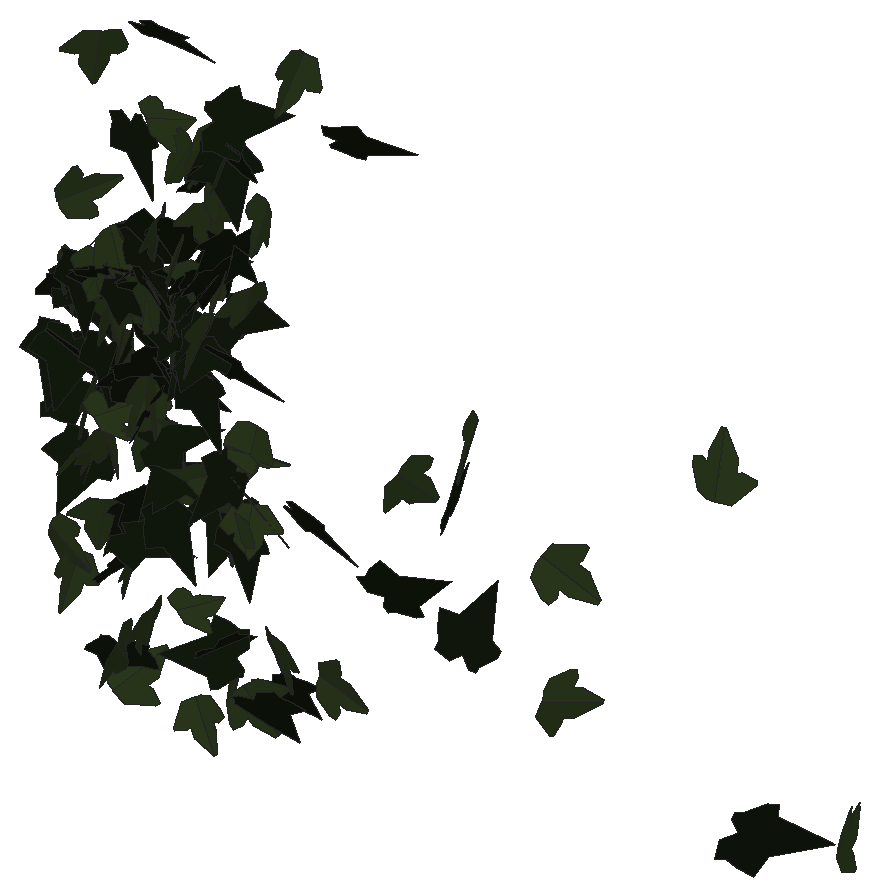
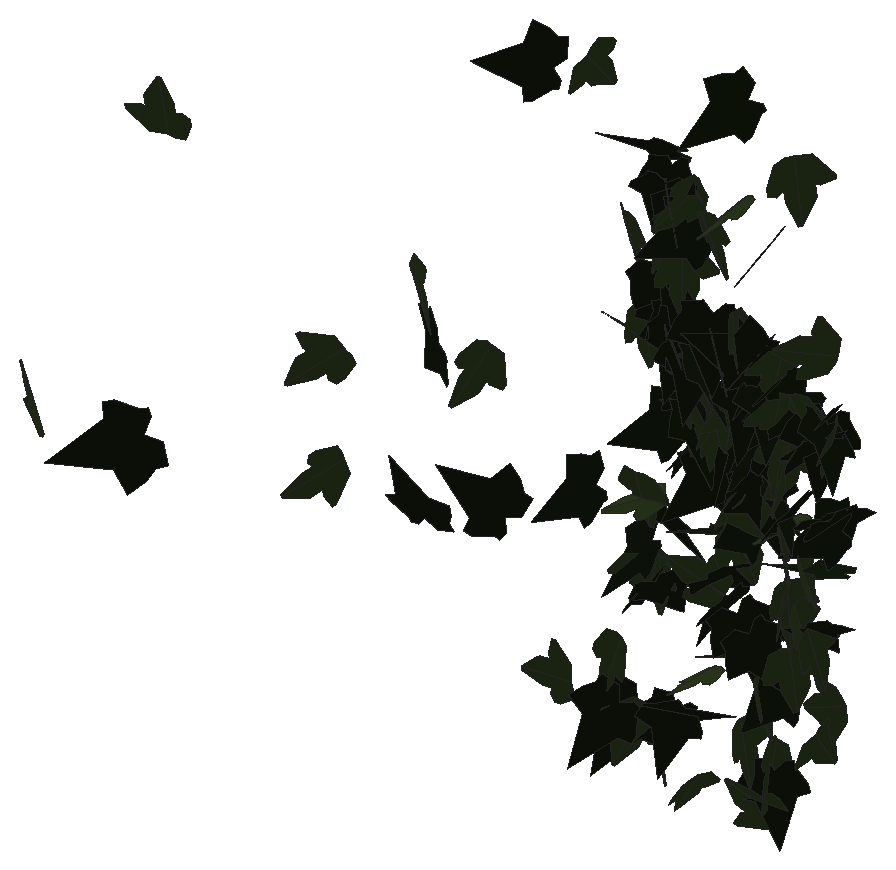
# SketchUp Ruby script. Lengths in inches.
U = 1.inch
M = Sketchup.active_model
def pt(a) = Geom::Point3d.new(a.map { |v| v * U })
def face(e, loops, mat)
  f = e.add_face(loops[0].map { |a| pt(a) })
  loops[1..].each { |l| e.add_face(l.map { |a| pt(a) }).erase! }
  f.material = f.back_material = mat if mat
  f
end
# faces: each face lists its corners as indices into pts; further lists are holes
def faces(e, pts, list, mat = nil) = list.each { |f| face(e, (f[0].is_a?(Array) ? f : [f]).map { |l| l.map { |i| pts[i] } }, mat) }
# xy, xz, yz: faces in a plane at the given z, y or x. An outline is a flat list of corners, or four numbers for a rectangle; further outlines are holes
def ring(l) = l.size == 4 ? [[l[0], l[1]], [l[2], l[1]], [l[2], l[3]], [l[0], l[3]]] : l.each_slice(2).to_a
def flat(e, list, mat, &to3) = list.each { |f| face(e, (f[0].is_a?(Array) ? f : [f]).map { |l| ring(l).map { |u, v| to3.(u, v) } }, mat) }
def xy(e, z, list, mat = nil) = flat(e, list, mat) { |x, y| [x, y, z] }
def xz(e, y, list, mat = nil) = flat(e, list, mat) { |x, z| [x, y, z] }
def yz(e, x, list, mat = nil) = flat(e, list, mat) { |y, z| [x, y, z] }
def lines(e, pts, list) = list.each { |a, b| e.add_line(pt(pts[a]), pt(pts[b])) }
# prism: a flat outline (further loops are holes) pulled along v
def prism(e, loops, v, mat = nil)
  f = face(e, loops, mat); d = Geom::Vector3d.new(v.map { |x| x * U })
  f.pushpull(f.normal.samedirection?(d) ? d.length : -d.length)
end
def box(e, o, s, mat = nil) = prism(e, [[o, [o[0] + s[0], o[1], o[2]], [o[0] + s[0], o[1] + s[1], o[2]], [o[0], o[1] + s[1], o[2]]]], [0, 0, s[2]], mat)
def at(x, y, z, deg = 0) = Geom::Transformation.translation(pt([x, y, z])) * Geom::Transformation.rotation(ORIGIN, Z_AXIS, deg.degrees)
def axes(o, x, y, z) = Geom::Transformation.new([*x, 0, *y, 0, *z, 0, *pt(o).to_a, 1])
def part(name) = M.definitions.add(name)
# library, detail: a bought-in or finely detailed component or shape, given as its bounding box
def library(name, o, s) = part(name).tap { |d| box(d.entities, o, s) }
def detail(e, o, s) = box(e.add_group.entities, o, s)
def put(e, d, t, mat = nil) = e.add_instance(d, t).tap { |i| i.material = mat if mat }
def group(e, t, mat = nil) = e.add_group.tap { |g| g.transformation = t; g.material = mat if mat }.entities
root = M.entities
M.materials.add("efeu1").color = [18, 25, 13]
M.materials.add("efeu2").color = [43, 57, 29]
c1 = part("ivyleaf_9")
p = [[1.54,2.16,1.25],[1.36,2.04,1.19],[-0.21,0.99,0.68],[-0.71,1.11,0.82],[-0.85,0.86,0.67],[-0.8,0.17,0.21],
  [-0.9,-0.01,0.1],[-0.67,-0.16,-0.02],[-0.08,-0.08,-0.05],[-0.03,-0.6,-0.4],[0.65,-0.88,-0.66],[0.83,-0.6,-0.49],
  [1.29,-0.42,-0.43],[1.8125,-0.07,-0.26],[1.21,0.44,0.15]]
faces(c1.entities,p,[[0,1,2,3,4,5,6,7,8,9,10,11,12,13,14]],"efeu1")
c2 = part("ivyleaf_10")
p = [[0,0.5,-0.03],[-0.0625,2.02,-0.43],[-0.19,2.01,-0.46],[-0.54,1.05,-0.29],[-0.52,0.625,-0.18],[-0.83,0.76,-0.28],
  [-1.16,0.64,-0.33],[-1.15,0.33,-0.24],[-0.77,-0.39,0.02],[-0.3,-0.51,0.16],[0.04,-0.48,0.23],[-0.02,2.01,-0.4375],
  [-0.06,2.01,-0.43],[0.04,-0.49,0.23],[0.67,-0.49,0.14],[1.38,0.36,-0.2],[1.375,0.51,-0.24],[0.81,0.65,-0.19],
  [0.62,0.59,-0.15],[0.6,1.09,-0.28],[0.5,1.23,-0.31]]
faces(c2.entities,p,[[0,1,2,3,4,5,6,7,8,9,10],[11,12,0,13,14,15,16,17,18,19,20]],"efeu2")
put(root,c1,axes([589.86,129.38,257.64],[-0.38156,-0.98328,-0.03529],[0.01021,0.03389,-1.05471],[0.98386,-0.38169,-0.00274]))
put(root,c1,axes([590.56,128.76,261.47],[-0.136,1.02686,0.32023],[-0.14631,0.30212,-1.03092],[-1.06564,-0.17253,0.10067]))
put(root,c2,axes([590.15,129.05,261.39],[-0.4513,0.99422,-0.05253],[-0.00038,-0.05785,-1.09158],[-0.9956,-0.45065,0.02423]))
put(root,c1,axes([589.49,129.37,257.3125],[1.00767,-0.24895,0.30361],[0.29888,-0.05592,-1.03783],[0.2546,1.05093,0.01669]))
put(root,c2,axes([590.42,129.98,252.09],[0.06529,-1.04507,0.14266],[0.00107,-0.14286,-1.04708],[1.05476,0.06483,-0.00777]))
put(root,c1,axes([590.3125,129.42,257.61],[-0.48859,-0.93303,-0.00792],[0.20269,-0.09741,-1.02896],[0.91078,-0.47885,0.22474]))
put(root,c1,axes([589.84,129,255.1],[0.95581,-0.42825,-0.09163],[0.37043,0.90792,-0.37927],[0.23362,0.31251,0.97629]))
put(root,c2,axes([590.58,129.38,247.28],[0.23753,0.84721,-0.56766],[-0.14143,-0.54986,-0.87982],[-1.00995,0.27625,-0.0103]))
put(root,c1,axes([590.76,129.91,252.54],[-0.71489,-0.78039,-0.02428],[0.12744,-0.08416,-1.04754],[0.7703,-0.71034,0.15078]))
put(root,c2,axes([590.11,128.87,248.73],[-0.43886,0.21107,-0.95915],[0.8493,-0.44597,-0.48674],[-0.49316,-0.95587,0.0153]))
put(root,c1,axes([590.99,128.35,261.39],[0.53183,0.9298,-0.32357],[-0.13362,-0.29619,-1.07074],[-0.97538,0.54755,-0.02974]))
put(root,c2,axes([590.9,129.92,255.37],[0.52404,-0.88255,0.26397],[0.14877,-0.21863,-1.02628],[0.90908,0.54451,0.01578]))
put(root,c2,axes([591.11,129.92,252.97],[0.28838,-1.01393,0.11412],[0.0212,-0.11261,-1.05409],[1.02011,0.28897,-0.01036]))
put(root,c2,axes([590.72,128.84,264.89],[-0.09538,-0.31554,1.0512],[0.34503,0.99305,0.32938],[-1.04189,0.35774,0.01285]))
put(root,c1,axes([590.61,129.5,261.02],[0.19183,-0.93138,-0.50614],[0.13029,0.53118,-0.92807],[1.05198,0.10405,0.20723]))
put(root,c1,axes([590.89,129.36,261.36],[0.16546,-1.04814,0.20582],[0.00088,-0.20814,-1.06066],[1.06815,0.16253,-0.03101]))
put(root,c2,axes([591.77,129.8,253.75],[-0.17683,-1.03716,-0.15633],[-0.01256,0.16062,-1.0514],[1.0488,-0.17295,-0.03895]))
put(root,c2,axes([592.03,129.375,250.38],[-0.75065,-0.73163,0.14522],[-0.08676,-0.11898,-1.04793],[0.74084,-0.75525,0.02442]))
put(root,c2,axes([592.0625,128.96,262.08],[1.00444,-0.14869,-0.34824],[-0.33329,0.12137,-1.01315],[0.17972,1.05614,0.0674]))
put(root,c2,axes([591.95,129.82,253.79],[-0.5981,0.87599,0.07694],[-0.0996,0.02497,-1.05852],[-0.87371,-0.60251,0.068]))
put(root,c2,axes([592.2,128.8125,272.86],[-0.69734,-0.89688,0.10443],[-0.06373,-0.08274,-1.13608],[0.90069,-0.70025,0.00047]))
put(root,c2,axes([592.05,129.91,256.5],[0.66885,-0.79938,-0.1908],[-0.03623,0.21709,-1.03651],[0.82104,0.66079,0.1097]))
put(root,c2,axes([592.07,129.59,259.75],[0.26078,-0.79806,-0.66927],[0.0487,0.69852,-0.81396],[1.04041,0.16733,0.20586]))
put(root,c2,axes([592.15,129.4,260.19],[-0.99073,-0.398,-0.15235],[0.13838,0.06422,-1.06766],[0.40307,-1.00032,-0.00792]))
put(root,c1,axes([591.73,129.96,257.57],[0.16584,-1.03842,0.11729],[0.01821,-0.11587,-1.05158],[1.04487,0.16683,-0.00029]))
put(root,c1,axes([592.75,129.2,257.4],[-0.29356,0.81079,0.61449],[-0.25433,0.56077,-0.86141],[-0.98504,-0.38642,0.03927]))
put(root,c1,axes([592.3,128.27,262.22],[0.93581,0.53696,0.15029],[-0.00478,0.30131,-1.04682],[-0.55757,0.89863,0.2612]))
put(root,c2,axes([592.52,129.59,262.08],[0.26357,1.03539,0.09613],[0.00661,0.0975,-1.06827],[-1.03982,0.26307,0.01758]))
put(root,c2,axes([592.73,129.82,258.26],[-0.31175,0.83029,-0.58184],[-0.10885,-0.63262,-0.84442],[-1.008,-0.18847,0.27113]))
put(root,c1,axes([593.27,128.85,244.49],[0.58049,0.6413,-0.62546],[-0.44201,-0.4432,-0.86466],[-0.77916,0.72921,0.02454]))
put(root,c1,axes([593.13,128.45,248.39],[0.43304,0.76397,0.62208],[0.13481,0.62718,-0.86407],[-0.97594,0.42562,0.15667]))
put(root,c1,axes([593.5,128.95,262.07],[0.01866,1.05808,0.18125],[-0.07109,0.1821,-1.0557],[-1.07113,0.00634,0.07323]))
put(root,c2,axes([593.1,128.69,263.77],[0.30685,1.0429,0.11688],[0.05005,0.10709,-1.08696],[-1.04823,0.3104,-0.01769]))
put(root,c2,axes([593.4,129.61,248.59],[0.4451,-0.99315,0.0222],[0.0073,-0.02105,-1.08832],[0.99337,0.44515,-0.00195]))
put(root,c2,axes([593.09,127.9,255.83],[0.90824,-0.21084,-0.51163],[0.28703,1.02019,0.08914],[0.4731,-0.2142,0.92812]))
put(root,c1,axes([593.74,129.79,251.09],[-0.08922,0.66953,-0.82047],[0.03161,-0.82133,-0.67367],[-1.05851,-0.08097,0.04904]))
put(root,c2,axes([593.72,128.16,244.92],[0.06981,-0.93094,-0.81556],[-0.03864,0.81482,-0.9334],[1.23705,0.07799,0.01687]))
put(root,c1,axes([594.04,128.88,257.85],[0.10411,0.93156,-0.55945],[-0.11503,-0.54941,-0.93624],[-1.08054,0.14824,0.04577]))
put(root,c1,axes([593.37,129.5,268.9],[0.43278,-1.03242,0.01485],[0.01332,-0.01052,-1.11943],[1.03244,0.43291,0.00821]))
put(root,c1,axes([593.56,128.34,262.14],[0.63344,-0.49743,-0.7037],[-0.28923,0.69998,-0.75515],[0.81177,0.63755,0.28005]))
put(root,c2,axes([593.28,129.17,242.73],[0.82898,0.01678,-0.80073],[0.77352,0.28198,0.80673],[0.20763,-1.11752,0.19153]))
put(root,c1,axes([594.47,129.66,251.73],[-0.02158,0.70195,-0.80631],[-0.22356,-0.7916,-0.68317],[-1.04541,0.1548,0.16274]))
put(root,c1,axes([594.27,128.93,262.04],[0.47618,0.98201,-0.12024],[-0.05841,-0.10531,-1.09135],[-0.98761,0.4797,0.00657]))
put(root,c2,axes([594.32,129.49,256.8],[0.21282,0.8897,-0.56607],[-0.27059,-0.51207,-0.90656],[-1.01921,0.32172,0.12248]))
put(root,c2,axes([594.46,129.34,246.18],[0.15815,-1.1246,-0.12054],[-0.01633,0.11943,-1.13567],[1.13093,0.15899,0.00046]))
put(root,c2,axes([594.76,128.74,261.65],[0.8528,-0.23315,-0.60781],[-0.51966,0.35952,-0.86704],[0.39209,0.98359,0.17284]))
put(root,c1,axes([593.91,129.45,263.74],[0.51669,-0.94339,-0.08218],[0.02789,0.10874,-1.0729],[0.94655,0.51176,0.07648]))
put(root,c1,axes([594.5,128.76,255.52],[0.20424,0.45591,0.94787],[0.23431,0.92159,-0.49376],[-1.02538,0.30141,0.07597]))
put(root,c1,axes([593.7,128.86,249.97],[0.77018,-0.5983,-0.32029],[0.38345,0.78338,-0.5413],[0.55992,0.28649,0.81126]))
put(root,c1,axes([593.875,129.73,259.28],[0.61037,-0.78535,0.386],[0.22284,-0.31562,-0.99451],[0.84624,0.64956,-0.01653]))
put(root,c2,axes([594.84,129.31,255.15],[-0.50119,-0.88341,0.35046],[-0.16255,-0.31069,-1.01561],[0.93638,-0.52677,0.01128]))
put(root,c1,axes([593.88,129.44,263.61],[0.29839,-0.01909,1.03753],[1.0377,0.00564,-0.29834],[-0.00014,1.07957,0.0199]))
put(root,c2,axes([594.875,129.35,264.93],[0.28665,-1.02814,-0.17905],[0.00028,0.18576,-1.06621],[1.04362,0.28235,0.04947]))
put(root,c1,axes([594.65,128.03,258.82],[0.63627,0.80949,0.29164],[0.17351,0.23455,-1.02959],[-0.84275,0.65945,0.00821]))
put(root,c2,axes([594.75,129.46,257.08],[-0.11871,1.02572,-0.30688],[-0.00604,-0.3094,-1.0318],[-1.07063,-0.11198,0.03985]))
put(root,c1,axes([594.21,129.3,262.25],[0.64468,-0.78764,0.37214],[0.24522,-0.28016,-1.01777],[0.8359,0.68965,0.01156]))
put(root,c2,axes([595.05,129.42,260.92],[0.23289,1.05288,-0.03205],[0.00761,-0.03451,-1.07822],[-1.05334,0.23254,-0.01487]))
put(root,c1,axes([595.53,130.21,253.35],[-0.63749,-0.81757,0.33916],[-0.08581,-0.35891,-1.02648],[0.88095,-0.62658,0.14544]))
put(root,c2,axes([595.17,128.78,270.15],[0.83002,-0.45389,-0.5865],[0.41148,1.0142,-0.20256],[0.617,-0.06576,0.92408]))
put(root,c2,axes([595.81,129.48,263.95],[0.5442,-0.9545,-0.19727],[-0.11299,0.16263,-1.0986],[0.9681,0.55553,-0.01732]))
put(root,c1,axes([596.54,128.64,260.75],[-0.66435,0.55926,0.64391],[-0.50518,0.39957,-0.86826],[-0.68715,-0.83446,0.01579]))
put(root,c1,axes([595.96,129.53,265.07],[0.55296,0.83088,-0.50179],[-0.29636,-0.4054,-0.99787],[-0.9243,0.62706,0.01976]))
put(root,c1,axes([595.28,128.26,274.78],[1.14558,0.16278,0.1317],[0.09828,0.22876,-1.13763],[-0.18489,1.13021,0.21129]))
put(root,c1,axes([595.27,128.54,254.96],[1.03088,-0.10607,-0.13824],[0.05689,0.98891,-0.33451],[0.1647,0.32231,0.98085]))
put(root,c2,axes([595.84,129.55,260.64],[-0.15609,0.94722,-0.52335],[-0.00575,-0.52948,-0.95661],[-1.08217,-0.13381,0.08057]))
put(root,c1,axes([596.56,129.7,263.0625],[-0.61041,0.92163,0.02249],[-0.01072,0.01987,-1.10544],[-0.92184,-0.6105,-0.00204]))
put(root,c1,axes([595.69,129.33,257.82],[0.98659,0.38759,0.22071],[0.20714,0.07633,-1.05998],[-0.39501,1.00809,-0.0046]))
put(root,c2,axes([596.46,129.14,268.99],[0.87187,-0.50726,-0.5025],[-0.40098,0.30837,-1.00702],[0.59079,0.9579,0.05809]))
put(root,c1,axes([595.79,128.75,251.73],[0.38674,-0.94924,-0.42474],[-0.12116,0.40894,-1.02427],[1.03285,0.40341,0.03889]))
put(root,c2,axes([595.84,129.96,259.99],[-0.75109,0.44988,-0.67449],[0.53903,-0.40971,-0.87353],[-0.60562,-0.92261,0.05902]))
put(root,c2,axes([596.72,129.94,262.76],[-0.86825,-0.47011,0.42813],[-0.27823,-0.37065,-0.97126],[0.57173,-0.8943,0.1775]))
put(root,c2,axes([595.76,129.75,252.7],[-0.46044,-0.28654,0.95842],[0.81933,0.49729,0.54229],[-0.57391,0.93983,0.00527]))
put(root,c1,axes([597.15,129.16,259.99],[-0.27669,1.04891,-0.09655],[-0.00008,-0.09984,-1.08449],[-1.05335,-0.27552,0.02544]))
put(root,c1,axes([596.9,129.375,263.13],[0.31106,1.0353,-0.02549],[-0.02598,-0.0188,-1.08084],[-1.03528,0.31154,0.01946]))
put(root,c1,axes([597.58,129.07,262.74],[-0.36059,1.02452,0.01335],[0.0002,0.01423,-1.08611],[-1.02461,-0.36056,-0.00491]))
put(root,c2,axes([596.98,128.57,247.71],[0.87411,-0.26946,-0.43016],[0.32721,0.954,0.06733],[0.38804,-0.19747,0.91222]))
put(root,c1,axes([597.61,129.32,260.46],[-0.87413,-0.64284,0.00344],[0.03426,-0.05239,-1.08326],[0.64194,-0.87257,0.0625]))
put(root,c2,axes([597.44,129.23,260.96],[0.30457,-0.90811,0.59404],[0.1965,-0.56064,-0.9578],[1.06721,0.36239,0.00682]))
put(root,c1,axes([597.66,129.16,263.75],[0.45734,0.9826,-0.02659],[-0.00263,-0.02811,-1.08378],[-0.98296,0.45725,-0.00947]))
put(root,c2,axes([597.19,129.15,242.78],[-0.24373,-0.95439,0.0326],[0.68216,-0.19755,-0.68335],[0.66827,-0.14643,0.70944]))
put(root,c1,axes([597.4,128.625,268.18],[0.59464,0.48775,0.77032],[0.42292,0.66719,-0.74892],[-0.80773,0.70841,0.17497]))
put(root,c2,axes([597.875,129.07,266.67],[-0.60854,-0.90255,-0.02439],[0.04721,-0.00243,-1.08779],[0.90164,-0.60903,0.0405]))
put(root,c1,axes([597.32,128.87,258.52],[0.38232,-0.99158,-0.21043],[-0.04554,0.20787,-1.06226],[1.01264,0.38371,0.03167]))
put(root,c2,axes([597.87,129.83,263.46],[0.74475,-0.77737,0.06495],[0.03691,-0.05458,-1.07649],[0.7792,0.74558,-0.01108]))
put(root,c1,axes([598.05,129.25,245.92],[0.34706,0.9378,0.03673],[0.01133,0.03497,-0.99996],[-0.93846,0.34724,0.00151]))
put(root,c1,axes([598.71,129.49,245.63],[-0.73584,0.10878,0.73853],[-0.73339,-0.29879,-0.68672],[0.13925,-0.99881,0.28586]))
put(root,c2,axes([597.74,128.58,269.71],[-0.09431,-0.48221,-0.99741],[0.44679,0.89945,-0.4771],[1.01378,-0.44126,0.11747]))
put(root,c1,axes([598.3,128.75,264.07],[-0.04488,1.04397,-0.27672],[0.03674,-0.27532,-1.04466],[-1.0794,-0.05278,-0.02405]))
put(root,c1,axes([598.1875,130.32,252.28],[-0.57501,-0.91712,-0.02718],[0.01183,0.02467,-1.08247],[0.91745,-0.57512,-0.00308]))
put(root,c1,axes([598.49,129.2,265.08],[0.67174,0.36495,-0.77532],[-0.69825,-0.33798,-0.76404],[-0.49675,0.96857,0.02553]))
put(root,c2,axes([598.5,128.65,268.16],[-0.02453,0.70818,0.84605],[-0.27524,0.81557,-0.69065],[-1.06843,-0.22636,0.1585]))
put(root,c2,axes([598.76,128.8,269.53],[0.46821,-0.9192,-0.36578],[-0.16941,0.3242,-1.03157],[0.97469,0.49791,-0.00359]))
put(root,c2,axes([598.83,129.48,244.7],[0.56229,-0.75033,-0.46469],[-0.22996,0.40741,-0.93608],[0.85209,0.60509,0.05403]))
put(root,c1,axes([597.9,129.46,259.4375],[1.01433,-0.20149,0.41978],[0.42431,-0.01439,-1.0322],[0.19175,1.09767,0.06353]))
put(root,c1,axes([599.13,129.02,254.72],[-1.03419,0.00523,-0.09638],[0.0965,0.03142,-1.03371],[-0.00229,-1.03819,-0.03177]))
put(root,c2,axes([599.01,129.27,252.24],[-0.98305,0.27873,0.12301],[-0.18153,-0.20212,-0.99267],[-0.24468,-0.96988,0.24222]))
put(root,c1,axes([599.29,128.89,265.93],[-0.14607,0.78644,-0.75317],[-0.11843,-0.76688,-0.77779],[-1.08247,-0.02222,0.18673]))
put(root,c1,axes([599.04,128.38,270.36],[0.82085,0.31762,-0.69178],[-0.6769,-0.16081,-0.87703],[-0.3482,1.06136,0.07414]))
put(root,c1,axes([598.9,128.8,269.84],[-0.5679,-0.59905,-0.72963],[0.47442,0.55505,-0.82497],[0.81618,-0.73945,-0.02815]))
put(root,c1,axes([599.06,129.72,251.68],[0.19469,-1.05131,0.07293],[0.00102,-0.07398,-1.06911],[1.05383,0.1943,-0.01244]))
put(root,c1,axes([598.6875,128.56,271.39],[0.96399,-0.33061,-0.44919],[0.36046,1.05376,-0.00201],[0.42561,-0.14364,1.01911]))
put(root,c1,axes([599.125,129.65,253.57],[1.05062,-0.28673,-0.22437],[-0.20451,0.10217,-1.08816],[0.30122,1.06944,0.0438]))
put(root,c2,axes([599.54,129.58,252.52],[0.76661,0.68682,-0.11772],[-0.08846,-0.07767,-1.02928],[-0.6912,0.7717,0.00117]))
put(root,c2,axes([599.56,129.69,256.2],[1.08445,-0.13951,-0.03035],[-0.0287,0.01473,-1.09333],[0.13986,1.08478,0.01095]))
put(root,c2,axes([599.2,129.34,255.48],[0.67361,-0.79265,0.0631],[0.79515,0.67113,-0.05779],[0.00332,0.0855,1.03861]))
put(root,c2,axes([600.04,128.81,263.45],[-0.2257,-1.07935,0.00265],[-0.00441,-0.00179,-1.10269],[1.07934,-0.22571,-0.00395]))
put(root,c1,axes([599.1,128.9,262.32],[0.62107,-0.79635,-0.35889],[0.82341,0.68072,-0.08553],[0.29149,-0.22616,1.00627]))
put(root,c2,axes([600.29,128.68,244.61],[0.67793,0.69075,0.63008],[0.1589,0.68184,-0.91846],[-0.92135,0.62585,0.30521]))
put(root,c2,axes([600.73,128.94,267.57],[0.89527,-0.61628,-0.14478],[-0.08039,0.13807,-1.08478],[0.62794,0.89633,0.06755]))
put(root,c1,axes([600.93,128.33,244.8],[0.99275,0.58947,-0.08514],[-0.07526,-0.04003,-1.15456],[-0.59081,0.99559,0.00399]))
put(root,c1,axes([601.02,129.4375,245.23],[0.9651,0.53396,0.01127],[0.00128,0.02097,-1.10282],[-0.53408,0.96494,0.01773]))
put(root,c2,axes([601.54,128.91,247.41],[-0.99448,0.54939,-0.06793],[0.06731,-0.01863,-1.13603],[-0.54947,-0.99662,-0.01621]))
put(root,c2,axes([602.24,129.54,274.82],[0.23658,0.85508,-0.69928],[-0.24253,-0.65748,-0.88602],[-1.07765,0.33569,0.04588]))
put(root,c1,axes([602.95,128.51,254.33],[1.10251,-0.21918,0.19676],[0.19524,-0.02693,-1.12403],[0.22053,1.1196,0.01148]))
put(root,c2,axes([603.4,129.91,245.82],[0.13939,-0.05489,1.12507],[1.11831,0.14239,-0.13161],[-0.13478,1.12469,0.07157]))
put(root,c1,axes([605.35,128.36,272.88],[0.76953,-0.17255,0.79377],[0.81125,0.10734,-0.76314],[0.04154,1.10033,0.19893]))
put(root,c1,axes([607.23,129.05,251.73],[0.17606,-0.22665,1.11858],[1.10977,-0.23021,-0.22132],[0.26642,1.1087,0.18271]))
put(root,c2,axes([608.74,128.32,258.14],[-0.3414,-0.77327,-0.80365],[0.40171,0.69878,-0.84302],[1.0404,-0.52355,0.06179]))
put(root,c1,axes([611.45,127.97,257.71],[0.01952,0.46169,1.12863],[-0.11504,1.12444,-0.45798],[-1.21397,-0.09913,0.06155]))
put(root,c1,axes([611.16,129.26,250.38],[-0.82163,0.38612,0.72618],[0.65951,-0.30397,0.90783],[0.4914,1.05357,-0.00422]))
put(root,c2,axes([611.75,128.95,261.09],[0.73485,-1.01341,0.00235],[0.00132,-0.00194,-1.2518],[1.01341,0.73485,-0.00008]))
put(root,c2,axes([615.9375,129.14,256.11],[0.48437,0.52661,0.95369],[0.6531,0.69501,-0.71547],[-0.87196,0.81309,-0.00611]))
put(root,c2,axes([616.5625,128.39,250.33],[-0.13818,-0.37024,-1.1162],[0.66108,0.90503,-0.38204],[0.9726,-0.66776,0.10109]))
put(root,c2,axes([625.08,128.6,263.39],[1.22231,0.15922,-0.02687],[0.02445,0.02037,1.23251],[0.15961,-1.22243,0.01703]))
put(root,c1,axes([626.97,127.875,247.91],[0.19536,0.41996,-1.27558],[0.30501,1.24145,0.45544],[1.30784,-0.35226,0.08433]))
put(root,c2,axes([631.01,129.54,247.96],[0.82186,-0.8309,-0.44817],[0.31624,-0.31757,1.16869],[-0.88952,-0.8806,0.00142]))
